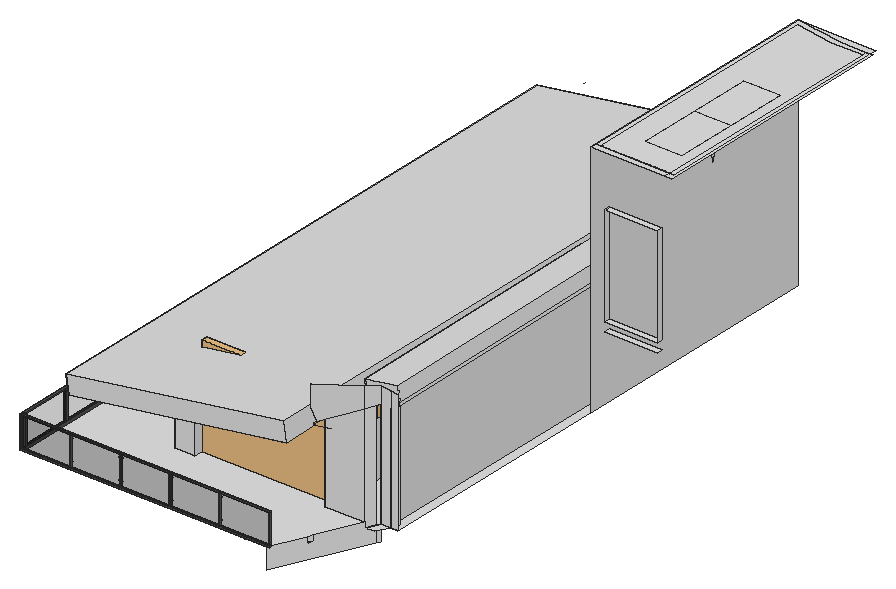
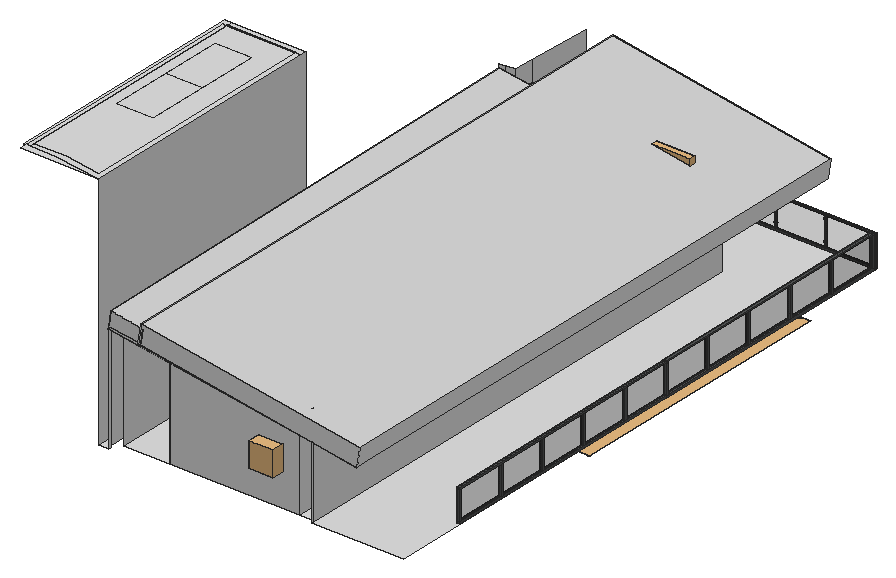
# SketchUp Ruby script. Lengths in inches.
U = 1.inch
M = Sketchup.active_model
def pt(a) = Geom::Point3d.new(a.map { |v| v * U })
def face(e, loops, mat)
  f = e.add_face(loops[0].map { |a| pt(a) })
  loops[1..].each { |l| e.add_face(l.map { |a| pt(a) }).erase! }
  f.material = f.back_material = mat if mat
  f
end
# faces: each face lists its corners as indices into pts; further lists are holes
def faces(e, pts, list, mat = nil) = list.each { |f| face(e, (f[0].is_a?(Array) ? f : [f]).map { |l| l.map { |i| pts[i] } }, mat) }
# xy, xz, yz: faces in a plane at the given z, y or x. An outline is a flat list of corners, or four numbers for a rectangle; further outlines are holes
def ring(l) = l.size == 4 ? [[l[0], l[1]], [l[2], l[1]], [l[2], l[3]], [l[0], l[3]]] : l.each_slice(2).to_a
def flat(e, list, mat, &to3) = list.each { |f| face(e, (f[0].is_a?(Array) ? f : [f]).map { |l| ring(l).map { |u, v| to3.(u, v) } }, mat) }
def xy(e, z, list, mat = nil) = flat(e, list, mat) { |x, y| [x, y, z] }
def xz(e, y, list, mat = nil) = flat(e, list, mat) { |x, z| [x, y, z] }
def yz(e, x, list, mat = nil) = flat(e, list, mat) { |y, z| [x, y, z] }
def lines(e, pts, list) = list.each { |a, b| e.add_line(pt(pts[a]), pt(pts[b])) }
# prism: a flat outline (further loops are holes) pulled along v
def prism(e, loops, v, mat = nil)
  f = face(e, loops, mat); d = Geom::Vector3d.new(v.map { |x| x * U })
  f.pushpull(f.normal.samedirection?(d) ? d.length : -d.length)
end
def box(e, o, s, mat = nil) = prism(e, [[o, [o[0] + s[0], o[1], o[2]], [o[0] + s[0], o[1] + s[1], o[2]], [o[0], o[1] + s[1], o[2]]]], [0, 0, s[2]], mat)
def at(x, y, z, deg = 0) = Geom::Transformation.translation(pt([x, y, z])) * Geom::Transformation.rotation(ORIGIN, Z_AXIS, deg.degrees)
def axes(o, x, y, z) = Geom::Transformation.new([*x, 0, *y, 0, *z, 0, *pt(o).to_a, 1])
def part(name) = M.definitions.add(name)
# library, detail: a bought-in or finely detailed component or shape, given as its bounding box
def library(name, o, s) = part(name).tap { |d| box(d.entities, o, s) }
def detail(e, o, s) = box(e.add_group.entities, o, s)
def put(e, d, t, mat = nil) = e.add_instance(d, t).tap { |i| i.material = mat if mat }
def group(e, t, mat = nil) = e.add_group.tap { |g| g.transformation = t; g.material = mat if mat }.entities
root = M.entities
M.materials.add("Aluminum_Polished").color = [83, 85, 85]
M.materials.add("Glass_Window_Neutral").color = [0, 0, 0]
M.materials["Glass_Window_Neutral"].alpha = 0.125
M.materials.add("[Color M03]").color = [226, 226, 226]
M.materials.add("[Wood Cherry Original]2").color = [152, 86, 42]
c1 = library("Mesh Light\#5",[-0.5,-0.5,-0.1],[1,1,0.2])
c2 = library("Mesh Light\#1",[-0.5,-0.5,-0.1],[1,1,0.2])
c3 = library("Group\#4",[-0.5,-0.5,-0.1],[66.16,13,0.2])
c4 = library("Sliding Door",[0,0,0],[94.49,5.83,91.73])
c5 = part("Group\#54")
box(c5.entities,[0,0,0],[2,1,28])
c6 = part("Group\#56")
p = [[0.11,0.32,0.14],[0.11,0.69,0.14]]
lines(c6.entities,p,[[0,1]])
g1 = group(c6.entities,at(0.11,0,0))
prism(g1,[[[0,0.24,0],[0,0.32,0.14],[0,0.24,0.27],[0,0.08,0.27],[0,0,0.14],[0,0.08,0]]],[-0.11,0,0])
c7 = part("Ver Glass Railing")
g2 = group(c7.entities,at(0,0,0),"Aluminum_Polished")
box(g2,[0,0,0],[2,185,2])
g3 = group(c7.entities,at(0,0,2),"Aluminum_Polished")
p = [[1.41,1,0],[1.41,36.8,0],[1.41,184,0],[1.29,184,0],[1.29,1,0],[1.29,36.8,0],
  [1.41,184,28],[1.29,184,28],[1.41,148.2,28],[1.29,148.2,28],[1.41,1,28],[1.29,1,28],
  [1.29,111.4,28],[1.29,111.4,0],[1.41,111.4,0],[1.41,111.4,28],[1.29,110.4,0],[1.29,110.4,28],
  [1.41,110.4,28],[1.41,110.4,0],[1.29,74.6,28],[1.29,74.6,0],[1.41,74.6,0],[1.41,74.6,28],
  [1.29,73.6,0],[1.29,73.6,28],[1.41,73.6,28],[1.41,73.6,0],[1.29,148.2,0],[1.41,148.2,0],
  [1.29,147.2,0],[1.29,147.2,28],[1.41,147.2,28],[1.41,147.2,0],[1.29,37.8,28],[1.29,37.8,0],
  [1.41,37.8,0],[1.41,37.8,28],[1.29,36.8,28],[1.41,36.8,28]]
lines(g3,p,[[0,1],[2,3],[4,5],[6,7],[6,8],[7,9],[10,11],[2,6],[3,7],[0,4],[11,4],[10,0],
  [12,13],[14,15],[16,17],[18,19],[20,21],[22,23],[24,25],[26,27],[27,22],[24,21],[23,26],[20,25],
  [9,28],[29,8],[30,31],[32,33],[33,29],[30,28],[8,32],[9,31],[34,35],[36,37],[5,38],[39,1],
  [1,36],[5,35],[37,39],[14,33],[19,14],[22,19],[36,27],[13,30],[16,13],[21,16],[35,24],[15,18],
  [12,17],[29,2],[28,3],[18,23],[32,15],[17,20],[31,12],[26,37],[25,34],[34,38],[39,10],[38,11]])
g4 = group(g3,at(1.79,1,0))
box(g4,[-0.5,0,0],[0.125,183,28],"Glass_Window_Neutral")
g5 = group(g3,at(0,184,28))
box(g5,[0,-184,0],[2.5,185,1])
put(g3,c5,axes([2,185,28],[-1,0,0],[0,-1,0],[0,0,-1]))
put(g3,c5,axes([2,1,28],[-1,0,0],[0,-1,0],[0,0,-1]))
put(g3,c5,axes([2,111.4,28],[-1,0,0],[0,-1,0],[0,0,-1]))
put(g3,c5,axes([2,74.6,28],[-1,0,0],[0,-1,0],[0,0,-1]))
g6 = group(g3,at(2,148.2,28))
box(g6,[-2,-1,-28],[2,1,28])
put(g3,c5,axes([2,37.8,28],[-1,0,0],[0,-1,0],[0,0,-1]))
put(g3,c6,at(1.17,146.31,24.26))
put(g3,c6,axes([1.17,148.89,24.54],[1,0,0],[0,-1,0],[0,0,-1]))
put(g3,c6,axes([1.17,148.89,4.79],[1,0,0],[0,-1,0],[0,0,-1]))
put(g3,c6,at(1.17,146.31,4.51))
put(g3,c6,at(1.17,109.51,4.51))
put(g3,c6,axes([1.17,112.09,4.79],[1,0,0],[0,-1,0],[0,0,-1]))
put(g3,c6,axes([1.17,112.09,24.54],[1,0,0],[0,-1,0],[0,0,-1]))
put(g3,c6,at(1.17,109.51,24.26))
put(g3,c6,axes([1.17,75.29,24.54],[1,0,0],[0,-1,0],[0,0,-1]))
put(g3,c6,at(1.17,72.71,4.51))
put(g3,c6,axes([1.17,75.29,4.79],[1,0,0],[0,-1,0],[0,0,-1]))
put(g3,c6,at(1.17,72.71,24.26))
put(g3,c6,axes([1.17,38.49,24.54],[1,0,0],[0,-1,0],[0,0,-1]))
put(g3,c6,at(1.17,35.91,4.51))
put(g3,c6,axes([1.17,38.49,4.79],[1,0,0],[0,-1,0],[0,0,-1]))
put(g3,c6,at(1.17,35.91,24.26))
c8 = part("Group257\#1")
p = [[0,0,0],[0,0,-16.65],[-7.38,0,-16.65],[48.07,-5.84,0],[-48.07,-5.84,0],[48.07,5.84,0],
  [48.07,0,0],[-48.07,5.84,0],[7.38,0,-16.65],[-48.07,0,0],[0,0,-26.95]]
lines(c8.entities,p,[[0,1],[1,2],[3,4],[5,6],[7,5],[1,8],[9,0],[0,6],[8,10],[4,9],[6,3],[2,10],
  [9,7]])
c9 = part("Rectangle Light")
put(c9.entities,c8,at(0,0,0))
c10 = library("Omni Light\#1",[-12,-12,-12],[24,24,24])
c11 = library("Mesh Light\#6",[-0.5,-0.5,-0.1],[1,1,0.2])
c12 = part("Group259\#1")
p = [[0,0,0],[0,0,-6.22],[-2.62,0,-6.22],[17.05,-3.08,0],[-17.05,-3.08,0],[17.05,3.08,0],
  [17.05,0,0],[-17.05,3.08,0],[2.62,0,-6.22],[-17.05,0,0],[0,0,-10.0625]]
lines(c12.entities,p,[[0,1],[1,2],[3,4],[5,6],[7,5],[1,8],[9,0],[0,6],[8,10],[4,9],[6,3],[2,10],
  [9,7]])
c13 = part("Rectangle Light\#1")
put(c13.entities,c12,at(0,0,0))
c14 = library("Omni Light",[-12,-12,-12],[24,24,24])
c15 = library("Group\#1",[-0.5,-0.5,0],[15.82,155.91,2.33])
c16 = library("Group\#5",[-0.5,-0.5,0],[12.84,12.98,1.86])
c17 = part("Group261\#1")
p = [[0,0,0],[0,0,-24.09],[-2.75,0,-24.09],[17.875,-60.125,0],[-17.875,-60.125,0],[17.875,60.125,0],
  [17.875,0,0],[-17.875,60.125,0],[2.75,0,-24.09],[-17.875,0,0],[0,0,-39]]
lines(c17.entities,p,[[0,1],[1,2],[3,4],[5,6],[7,5],[1,8],[9,0],[0,6],[8,10],[4,9],[6,3],[2,10],
  [9,7]])
c18 = part("Rectangle Light\#2")
put(c18.entities,c17,at(0,0,0))
xy(root,328.48,[[507.65,174.67,509.43,174.67,509.43,178.59],[528.06,219.62,537.125,219.62,542.76,232.04,533.7,232.04,533.7,227.88,531.81,227.88],[350.6,227.88,361.96,709.81],[361.96,227.88,489.14,709.81],[489.14,227.88,531.81,227.88,533.7,232.04,533.7,709.81,489.14,709.81],
  [531.81,227.88,533.7,227.88,533.7,232.04],[542.76,232.04,550.5,232.04,550.5,720.04,540.65,720.04,540.62,718.0625,541.95,718.0625,541.95,239.77,546.15,239.49]],"[Color M03]")
xy(root,333.29,[[252.37,143.16,493.34,143.16,507.65,174.67,509.43,178.59,528.06,219.62,489.14,219.62,489.14,227.88,361.96,227.88,361.96,219.62,342.34,219.62,342.34,720.04,252.37,720.04]],"[Color M03]")
xy(root,404.08,[[564.58,466.93,616.16,472.23]],"[Color M03]")
xy(root,412.95,[[564.45,466.93,616.16,472.23]],"[Color M03]")
xy(root,432.98,[[528.06,219.62,531.81,227.88,528.06,227.88]],"[Color M03]")
xy(root,510.7,[[564.45,466.93,616.16,472.23]],"[Color M03]")
xy(root,561.04,[[550.5,466.93,622.99,466.93,622.99,472.23,555.8,472.23,555.8,473.1,550.5,473.1],[622.99,466.93,629.37,466.93,629.37,712.68,627.06,712.68,627.06,473.1,623.13,473.1,623.13,472.23,622.99,472.23],[555.8,472.23,622.99,473.1],[622.99,472.23,623.13,473.1],[550.5,473.1,555.8,473.1,555.8,713.83,591.7,708.16,622.99,708.16,622.99,712.68,597,712.68,550.5,720.04],
  [555.8,473.1,622.99,473.1,622.99,708.16,591.7,708.16,555.8,713.83],[622.99,473.1,623.13,708.16],[623.13,473.1,627.06,473.1,627.06,712.68,622.99,712.68,622.99,708.16,623.13,708.16],[597,712.68,627.06,712.68,627.06,720.04,550.5,720.04]],"[Color M03]")
xz(root,144.37,[[298.69,396.87,511.89,430.43,509.06,448.4,295.86,414.83]],"[Color M03]")
xz(root,219.62,[[342.34,333.29,361.96,333.29,361.96,406.83,342.34,403.74],[489.14,333.29,528.06,333.29,528.06,432.98,509.91,430.125,489.14,426.85]],"[Color M03]")
xz(root,227.88,[[350.6,328.48,350.6,405.04,361.96,406.83,361.96,328.48],[361.96,328.48,489.14,333.29],[489.14,328.48,489.14,426.85,509.91,430.125,528.06,432.98,531.81,432.98,531.81,328.48]],"[Color M03]")
xz(root,232.04,[[533.7,328.48,533.7,449.22,542.76,448.11,542.76,328.48],[542.76,328.48,542.76,448.11,550.5,447.16,550.5,328.48]],"[Color M03]")
xz(root,709.81,[[361.96,328.48,489.14,328.48,489.14,426.85,361.96,406.83]],"[Color M03]")
xz(root,718.0625,[[540.62,328.48,541.95,432.98]],"[Color M03]")
xz(root,720.04,[[298.69,396.87,295.86,414.83,509.06,448.4,511.89,430.43,342.34,403.74]],"[Color M03]")
yz(root,342.34,[[219.62,333.29,718.0625,403.74],[718.0625,333.29,720.04,403.74]],"[Color M03]")
yz(root,350.6,[[227.88,328.48,709.81,405.04]],"[Color M03]")
yz(root,361.96,[[227.88,328.48,709.81,406.83],[219.62,333.29,227.88,404.86],[219.62,404.86,227.88,406.83]],"[Color M03]")
yz(root,489.14,[[227.88,328.48,709.81,426.85],[219.62,333.29,227.88,426.85]],"[Color M03]")
yz(root,533.7,[[232.04,328.48,709.81,432.98]],"[Color M03]")
yz(root,541.95,[[239.77,328.48,718.0625,432.98]],"[Color M03]")
yz(root,550.5,[[466.93,328.48,720.04,561.04]],"[Color M03]")
yz(root,564.45,[[466.93,412.95,472.23,510.7]],"[Color M03]")
yz(root,616.16,[[466.93,412.95,472.23,510.7]],"[Color M03]")
p = [[493.34,143.16,312.98],[531.81,227.88,312.98],[531.81,227.88,328.48],[528.06,219.62,328.48],[528.06,219.62,333.29],[509.43,178.59,333.29],
  [509.43,178.59,328.48],[507.65,174.67,328.48],[507.65,174.67,333.29],[493.34,143.16,333.29],[533.7,232.04,328.48],[533.7,232.04,312.98],
  [531.81,227.88,432.98],[528.06,219.62,432.98],[542.76,232.04,328.48],[546.15,239.49,328.48],[546.15,239.49,432.98],[542.76,232.04,432.98],
  [541.95,239.77,328.48],[541.95,239.77,432.98],[540.62,718.0625,328.48],[540.65,720.04,328.48],[540.65,720.04,432.98],[540.62,718.0625,432.98],
  [298.69,709.81,396.87],[298.69,144.37,396.87],[295.86,144.37,414.83],[295.86,720.04,414.83],[298.69,720.04,396.87],[298.69,718.0625,396.87],
  [342.34,709.81,403.74],[342.34,219.62,403.74],[361.96,219.62,406.83],[361.96,227.88,406.83],[361.96,709.81,406.83],[489.14,709.81,426.85],
  [489.14,227.88,426.85],[489.14,219.62,426.85],[509.91,219.62,430.125],[509.91,219.01,430.125],[509.91,178.79,430.125],[511.89,178.79,430.43],
  [511.89,144.37,430.43],[427.58,317.46,417.16],[428.52,318.7,417.31],[429.11,320.15,417.4],[429.3125,321.7,417.43],[429.11,323.26,417.4],
  [428.52,324.7,417.31],[427.58,325.95,417.16],[426.35,326.9,416.97],[424.92,327.5,416.74],[423.39,327.7,416.5],[421.85,327.5,416.26],
  [420.42,326.9,416.03],[419.2,325.95,415.84],[418.25,324.7,415.69],[417.66,323.26,415.6],[417.46,321.7,415.57],[417.66,320.15,415.6],
  [418.25,318.7,415.69],[419.2,317.46,415.84],[420.42,316.51,416.03],[421.85,315.91,416.26],[423.39,315.7,416.5],[424.92,315.91,416.74],
  [426.35,316.51,416.97],[426.36,470.61,416.97],[424.82,470.4,416.73],[423.39,469.81,416.5],[422.17,468.85,416.31],[421.22,467.61,416.16],
  [420.63,466.16,416.07],[420.43,464.61,416.03],[420.63,463.06,416.07],[421.22,461.61,416.16],[422.17,460.37,416.31],[423.39,459.41,416.5],
  [424.82,458.8125,416.73],[426.36,458.61,416.97],[427.89,458.8125,417.21],[429.32,459.41,417.43],[430.55,460.37,417.63],[431.49,461.61,417.78],
  [432.08,463.06,417.87],[432.28,464.61,417.9],[432.08,466.16,417.87],[431.49,467.61,417.78],[430.55,468.85,417.63],[429.32,469.81,417.43],
  [427.89,470.4,417.21],[427.66,399.28,417.17],[428.88,400.23,417.37],[429.83,401.47,417.51],[430.42,402.92,417.61],[430.62,404.47,417.64],
  [430.42,406.03,417.61],[429.83,407.47,417.51],[428.88,408.72,417.37],[427.66,409.67,417.17],[426.23,410.27,416.95],[424.69,410.47,416.71],
  [423.16,410.27,416.46],[421.73,409.67,416.24],[420.5,408.72,416.05],[419.56,407.47,415.9],[418.97,406.03,415.8],[418.77,404.47,415.77],
  [418.97,402.92,415.8],[419.56,401.47,415.9],[420.5,400.23,416.05],[421.73,399.28,416.24],[423.16,398.68,416.46],[424.69,398.47,416.71],
  [426.23,398.68,416.95],[450.32,163.72,420.74],[450.61,165.26,420.79],[450.49,166.82,420.77],[449.97,168.3,420.69],[449.1,169.59,420.55],
  [447.92,170.61,420.36],[446.52,171.28,420.14],[445,171.57,419.9],[443.46,171.45,419.66],[442,170.93,419.43],[440.73,170.04,419.23],
  [439.72,168.85,419.07],[439.05,167.4375,418.97],[438.77,165.9,418.92],[438.89,164.34,418.94],[439.4,162.86,419.02],[440.28,161.57,419.16],
  [441.45,160.55,419.34],[442.85,159.87,419.5625],[444.37,159.59,419.8],[445.91,159.71,420.05],[447.375,160.23,420.28],[448.65,161.11,420.48],
  [449.66,162.31,420.64],[342.34,718.0625,403.74],[342.34,720.04,403.74],[350.6,227.88,405.04],[350.6,709.81,405.04],[511.89,720.04,430.43],
  [511.89,541.08,430.43],[509.91,541.08,430.125],[509.91,239.18,430.125],[509.91,227.88,430.125],[509.91,719.73,428.45],[509.06,720.04,448.4],
  [509.06,144.37,448.4],[417.55,320.15,416.34],[418.14,318.7,416.43],[417.34,321.7,416.31],[417.55,323.26,416.34],[418.14,324.7,416.43],
  [419.08,317.46,416.58],[419.08,325.95,416.58],[420.31,316.51,416.77],[420.31,326.9,416.77],[418.85,402.92,416.54],[419.44,401.47,416.64],
  [418.65,404.47,416.51],[418.85,406.03,416.54],[419.44,407.47,416.64],[420.38,400.23,416.79],[420.38,408.72,416.79],[421.74,315.91,417],
  [421.74,327.5,417],[421.61,399.28,416.98],[421.61,409.67,416.98],[420.3125,464.61,416.78],[420.51,463.06,416.81],[420.51,466.16,416.81],
  [421.11,461.61,416.9],[421.11,467.61,416.9],[423.04,398.68,417.2],[423.04,410.27,417.2],[422.05,460.37,417.05],[422.05,468.85,417.05],
  [423.27,315.7,417.24],[423.27,327.7,417.24],[423.28,459.41,417.24],[423.28,469.81,417.24],[424.8,315.91,417.48],[424.8,327.5,417.48],
  [424.58,398.47,417.45],[424.58,410.47,417.45],[424.71,458.8125,417.47],[424.71,470.4,417.47],[426.23,316.51,417.71],[426.23,326.9,417.71],
  [426.11,398.68,417.6875],[426.11,410.27,417.6875],[426.24,458.61,417.71],[426.24,470.61,417.71],[427.54,399.28,417.91],[427.54,409.67,417.91],
  [427.46,317.46,417.9],[427.46,325.95,417.9],[427.77,458.8125,417.95],[427.77,470.4,417.95],[428.4,318.7,418.05],[428.4,324.7,418.05],
  [428.77,400.23,418.11],[428.77,408.72,418.11],[429.2,459.41,418.17],[429.2,469.81,418.17],[429,320.15,418.14],[429,323.26,418.14],
  [429.2,321.7,418.17],[429.71,401.47,418.25],[429.71,407.47,418.25],[430.43,460.37,418.37],[430.43,468.85,418.37],[430.3,402.92,418.35],
  [430.3,406.03,418.35],[430.5,404.47,418.38],[431.37,461.61,418.52],[431.37,467.61,418.52],[431.96,463.06,418.61],[431.96,466.16,418.61],
  [432.17,464.61,418.64],[438.6,164.34,420.79],[439.11,162.86,420.875],[438.48,165.9,420.77],[438.76,167.4375,420.82],[439.99,161.57,421.01],
  [439.43,168.85,420.92],[440.43,170.04,421.08],[441.16,160.55,421.2],[441.71,170.93,421.28],[442.56,159.87,421.42],[443.17,171.45,421.51],
  [444.08,159.59,421.66],[444.71,171.57,421.76],[445.62,159.71,421.9],[446.23,171.28,421.99],[447.08,160.23,422.13],[447.63,170.61,422.21],
  [448.36,161.11,422.33],[448.8,169.59,422.4],[449.36,162.31,422.49],[449.68,168.3,422.54],[450.03,163.72,422.59],[450.3125,165.26,422.64],
  [450.19,166.82,422.62],[514.72,239.18,428.35],[514.43,239.17,430.32],[509.62,719.73,430.43],[541.34,720.05,433.08],[514.72,541.08,428.35],
  [545.86,239.49,434.96],[540.36,720.03,434.96],[509.46,176.05,432.98],[533.7,232.04,432.98],[528.06,219.01,432.98],[511.4375,176.05,433.29],
  [511.89,239.18,430.43],[528.06,227.88,432.98],[512.27,239.15,444.92],[507.47,719.7,445.02],[543.71,239.46,449.55],[541.05,720.04,435.0625],
  [538.2,720.01,449.55],[509.46,176.05,466.59],[528.06,219.01,453.26],[533.7,232.04,449.22],[538.9,720.02,449.65],[308.8,233.64,328.48],
  [308.8,239.64,328.48],[342.34,718.0625,432.98],[342.34,720.04,432.98],[528.06,178.79,432.98],[361.96,223.32,405.75],[489.14,222.9375,424.78]]
faces(root,p,[[0,1,2,3,4,5,6,7,8,9],[10,2,1,11],[7,6,5,8],[3,2,12,13,4],[14,15,16,17],[15,18,19,16],[20,21,22,23],[24,25,26,27,28,29],
  [139,30,24,29],[140,139,29,28],[141,33,32,31,30,142],[140,143,144,145,146,147,36,35,34,33,141,142,30,139],[22,140,139,148],[149,27,26,150],[60,59,151,152],[59,58,153,151],
  [58,57,154,153],[57,56,155,154],[61,60,152,156],[56,55,157,155],[62,61,156,158],[55,54,159,157],[109,108,160,161],[108,107,162,160],
  [107,106,163,162],[106,105,164,163],[110,109,161,165],[105,104,166,164],[63,62,158,167],[54,53,168,159],[111,110,165,169],[104,103,170,166],
  [74,73,171,172],[73,72,173,171],[75,74,172,174],[72,71,175,173],[112,111,169,176],[103,102,177,170],[76,75,174,178],[71,70,179,175],
  [64,63,167,180],[53,52,181,168],[77,76,178,182],[70,69,183,179],[65,64,180,184],[52,51,185,181],[113,112,176,186],[102,101,187,177],
  [78,77,182,188],[69,68,189,183],[66,65,184,190],[51,50,191,185],[114,113,186,192],[101,100,193,187],[79,78,188,194],[68,67,195,189],
  [91,114,192,196],[100,99,197,193],[43,66,190,198],[50,49,199,191],[80,79,194,200],[67,90,201,195],[44,43,198,202],[49,48,203,199],
  [92,91,196,204],[99,98,205,197],[81,80,200,206],[90,89,207,201],[45,44,202,208],[48,47,209,203],[46,45,208,210],[47,46,210,209],
  [93,92,204,211],[98,97,212,205],[82,81,206,213],[89,88,214,207],[94,93,211,215],[97,96,216,212],[95,94,215,217],[96,95,217,216],
  [83,82,213,218],[88,87,219,214],[84,83,218,220],[87,86,221,219],[85,84,220,222],[86,85,222,221],[130,129,223,224],[129,128,225,223],
  [128,127,226,225],[131,130,224,227],[127,126,228,226],[126,125,229,228],[132,131,227,230],[125,124,231,229],[133,132,230,232],[124,123,233,231],
  [134,133,232,234],[123,122,235,233],[135,134,234,236],[122,121,237,235],[136,135,236,238],[121,120,239,237],[137,136,238,240],[120,119,241,239],
  [138,137,240,242],[119,118,243,241],[115,138,242,244],[116,115,244,245],[118,117,246,243],[117,116,245,246],[37,36,147,38],[148,247,248,249],
  [16,247,148,22,250],[251,247,146,145],[247,16,252,248],[22,148,249,253],[147,146,254,40,39,38],[255,146,254,256],[40,254,257,41],[254,146,258,257],
  [259,13,38,147],[146,145,144,258],[249,248,260,261],[248,252,262,260],[252,248,249,253,263],[42,41,257,258,144,143,149,150],[253,249,261,264],[254,265,266,256],
  [256,266,267,255],[16,250,263,252],[250,22,253,263],[252,263,268,262],[263,253,264,268],[260,262,268,264,261]],"[Color M03]")
faces(root,p,[[[30,31,32,33,34,35,36,37,38,39,40,41,42,25,24],[43,44,45,46,47,48,49,50,51,52,53,54,55,56,57,58,59,60,61,62,63,64,65,66],[67,68,69,70,71,72,73,74,75,76,77,78,79,80,81,82,83,84,85,86,87,88,89,90],[91,92,93,94,95,96,97,98,99,100,101,102,103,104,105,106,107,108,109,110,111,112,113,114],[115,116,117,118,119,120,121,122,123,124,125,126,127,128,129,130,131,132,133,134,135,136,137,138]]],"[Wood Cherry Original]2")
lines(root,p,[[269,270],[271,272],[273,41],[256,39],[274,275]])
g7 = group(root,at(269.74,202.57,308.04),"[Color M03]")
xy(g7,0,[[6.52,0,4.95,0.07,3.46,0.54,2.14,1.38,1.08,2.54,0.36,3.93,0.02,5.46,0.09,7.02,0.5625,8.52,1.41,9.84,2.5625,10.9,3.95,11.62,5.48,11.96,7.05,11.89,8.54,11.41,9.86,10.57,10.92,9.41,11.64,8.02,11.98,6.5,11.91,4.93,11.4375,3.4375,10.59,2.12,9.4375,1.06,8.05,0.34],[6,123.04,4.45,123.24,3,123.84,1.76,124.8,0.8,126.04,0.2,127.48,0,129.04,0.2,130.59,0.8,132.04,1.76,133.28,3,134.23,4.45,134.83,6,135.04,7.55,134.83,9,134.23,10.24,133.28,11.2,132.04,11.8,130.59,12,129.04,11.8,127.48,11.2,126.04,10.24,124.8,9,123.84,7.55,123.24],[6,256.57,4.45,256.78,3,257.38,1.76,258.33,0.8,259.57,0.2,261.02,0,262.57,0.2,264.125,0.8,265.57,1.76,266.82,3,267.77,4.45,268.37,6,268.57,7.55,268.37,9,267.77,10.24,266.82,11.2,265.57,11.8,264.125,12,262.57,11.8,261.02,11.2,259.57,10.24,258.33,9,257.38,7.55,256.78]])
put(g7,c1,axes([6,134.29,0],[13,0,0],[0,269.57394,0],[0,0,1]))
g8 = group(root,at(436.84,328.26,308.17),"[Color M03]")
xy(g8,0,[[6,0,5.02,0.13,4.1,0.51,3.3125,1.11,2.71,1.9,2.33,2.82,2.2,3.8,2.33,4.78,2.71,5.7,3.3125,6.49,4.1,7.09,5.02,7.47,6,7.6,6.98,7.47,7.9,7.09,8.6875,6.49,9.29,5.7,9.67,4.78,9.8,3.8,9.67,2.82,9.29,1.9,8.6875,1.11,7.9,0.51,6.98,0.13],[6,25.85,4.45,26.06,3,26.66,1.76,27.61,0.8,28.85,0.2,30.3,0,31.85,0.2,33.41,0.8,34.85,1.76,36.1,3,37.05,4.45,37.65,6,37.85,7.55,37.65,9,37.05,10.24,36.1,11.2,34.85,11.8,33.41,12,31.85,11.8,30.3,11.2,28.85,10.24,27.61,9,26.66,7.55,26.06],[6,85.09,5.11,85.2,4.28,85.55,3.57,86.09,3.02,86.81,2.68,87.64,2.5625,88.53,2.68,89.41,3.02,90.24,3.57,90.96,4.28,91.5,5.11,91.85,6,91.96,6.89,91.85,7.72,91.5,8.43,90.96,8.98,90.24,9.32,89.41,9.4375,88.53,9.32,87.64,8.98,86.81,8.43,86.09,7.72,85.55,6.89,85.2],[6,139.56,4.45,139.76,3,140.36,1.76,141.32,0.8,142.56,0.2,144.01,0,145.56,0.2,147.11,0.8,148.56,1.76,149.8,3,150.75,4.45,151.35,6,151.56,7.55,151.35,9,150.75,10.24,149.8,11.2,148.56,11.8,147.11,12,145.56,11.8,144.01,11.2,142.56,10.24,141.32,9,140.36,7.55,139.76],[6,201.24,4.45,201.44,3,202.04,1.76,202.99,0.8,204.24,0.2,205.68,0,207.24,0.2,208.79,0.8,210.24,1.76,211.48,3,212.43,4.45,213.03,6,213.24,7.55,213.03,9,212.43,10.24,211.48,11.2,210.24,11.8,208.79,12,207.24,11.8,205.68,11.2,204.24,10.24,202.99,9,202.04,7.55,201.44]])
put(g8,c2,axes([6,106.62,0],[13,0,0],[0,214.23741,0],[0,0,1]))
put(root,c3,at(380.3125,177.38,308.86),"[Color M03]")
put(root,c4,axes([361.96,227.88,328.48],[1.34602,0,0],[0,1,0],[0,0,1.12]),"[Color M03]")
put(root,c7,axes([252.37,397.98,333.29],[1.37,0,0],[0,1.37,0],[0,0,1.0138]),"[Color M03]")
put(root,c7,axes([252.37,145.9,333.29],[1.37,0,0],[0,1.37,0],[0,0,1.0412]),"[Color M03]")
put(root,c7,axes([496.15,143.16,333.29],[0,0.5891,0],[-1.31773,0,0],[0,0,1.0275]),"[Color M03]")
put(root,c9,axes([489.13,509.94,361.66],[0,-2.2936,0],[0,0,-2.2936],[2.2936,0,0]))
put(root,c10,at(390.73,709.81,372.72))
g9 = group(root,at(489.14,709.81,383.1))
yz(g9,0,[[-425.25,0,0,11.0625]],"[Color M03]")
put(g9,c11,axes([0,-212.625,5.53],[0,-426.25,0],[0,0,12.0625],[-1,0,0]))
put(root,c13,axes([435.62,558.15,410.25],[2.37,0,0],[0,2.37,0],[0,0,2.37]))
put(root,c14,at(424.69,410.47,416.71))
put(root,c15,at(417.34,315.7,416.31),"[Color M03]")
put(root,c16,at(438.48,159.59,420.77),"[Color M03]")
put(root,c18,at(595.27,559.93,561.03))
